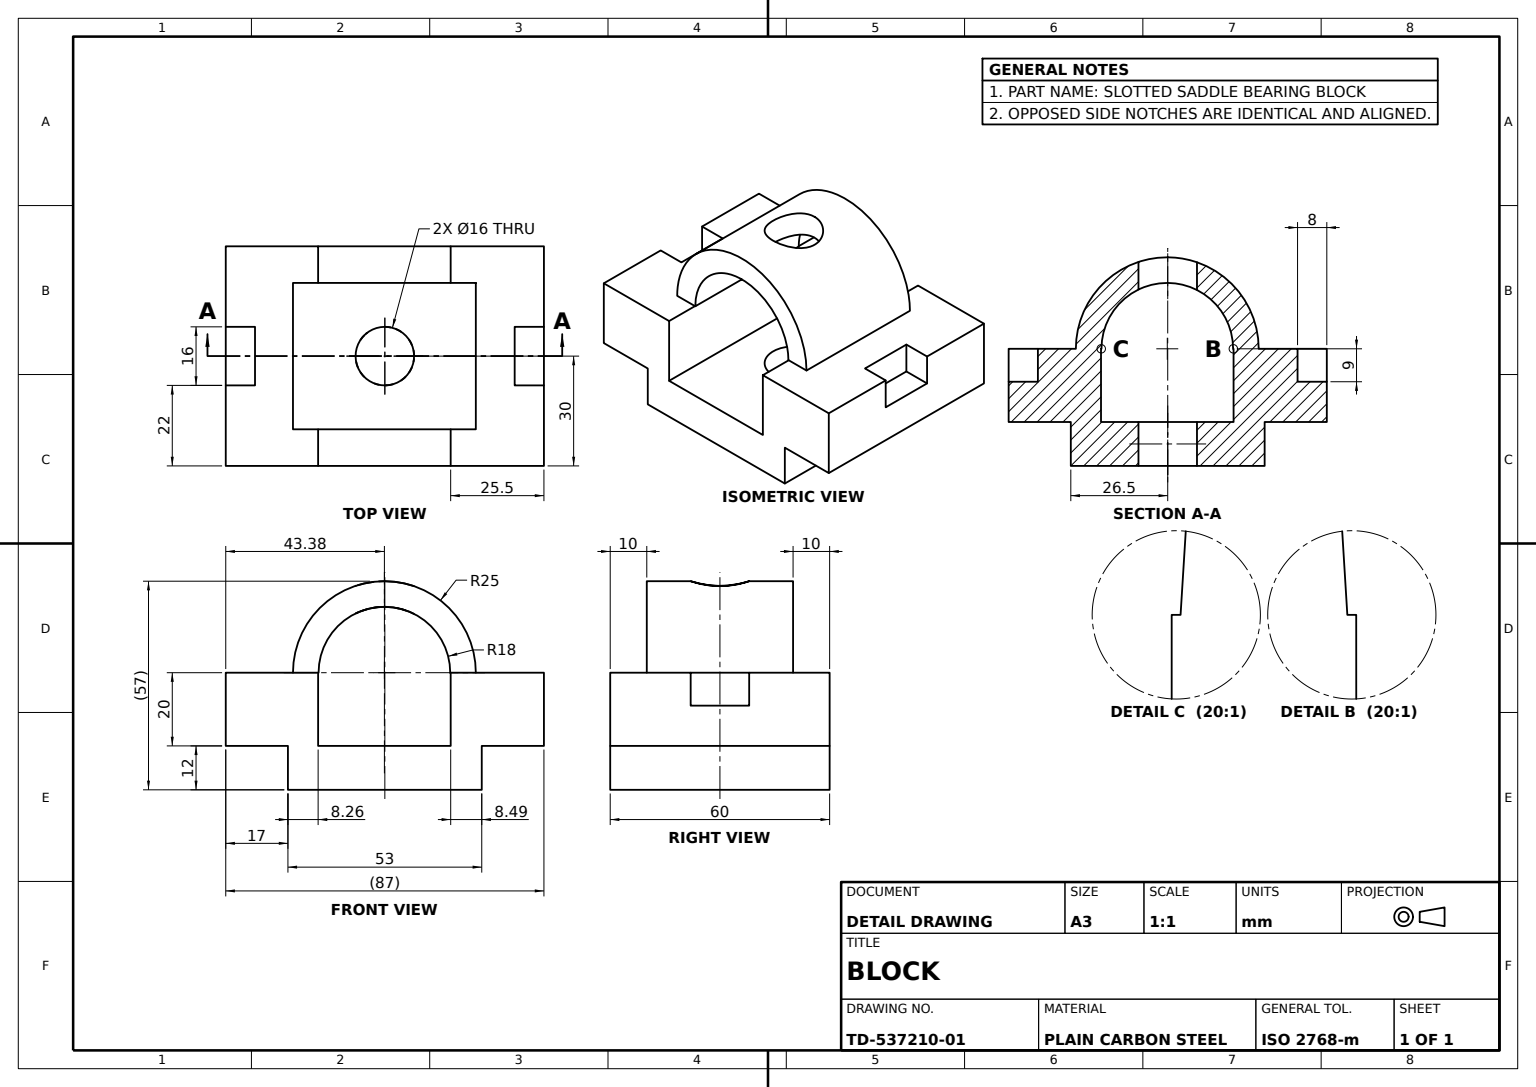
ISO-10303-21;
HEADER;
FILE_DESCRIPTION((''),'2;1');
FILE_NAME('','',(''),(''),'','','');
FILE_SCHEMA(('AUTOMOTIVE_DESIGN'));
ENDSEC;
DATA;
#1=APPLICATION_CONTEXT('');
#2=PRODUCT_CONTEXT('',#1,'mechanical');
#3=PRODUCT('','','',(#2));
#4=PRODUCT_DEFINITION_FORMATION('','',#3);
#5=PRODUCT_DEFINITION_CONTEXT('',#1,'design');
#6=PRODUCT_DEFINITION('','',#4,#5);
#7=PRODUCT_DEFINITION_SHAPE('','',#6);
#8=(LENGTH_UNIT()NAMED_UNIT(*)SI_UNIT(.MILLI.,.METRE.));
#9=(NAMED_UNIT(*)PLANE_ANGLE_UNIT()SI_UNIT($,.RADIAN.));
#10=(NAMED_UNIT(*)SI_UNIT($,.STERADIAN.)SOLID_ANGLE_UNIT());
#11=UNCERTAINTY_MEASURE_WITH_UNIT(LENGTH_MEASURE(1.E-05),#8,'distance_accuracy_value','');
#12=(GEOMETRIC_REPRESENTATION_CONTEXT(3)GLOBAL_UNCERTAINTY_ASSIGNED_CONTEXT((#11))GLOBAL_UNIT_ASSIGNED_CONTEXT((#8,#9,#10))REPRESENTATION_CONTEXT('',''));
#13=CARTESIAN_POINT('',(8.37856,32.,-10.));
#14=VERTEX_POINT('',#13);
#15=CARTESIAN_POINT('',(44.37856,32.,-10.));
#16=VERTEX_POINT('',#15);
#17=CARTESIAN_POINT('',(26.37856,32.,-10.));
#18=DIRECTION('',(0.,0.,-1.));
#19=DIRECTION('',(1.,0.,0.));
#20=AXIS2_PLACEMENT_3D('',#17,#18,#19);
#21=CIRCLE('',#20,18.);
#22=EDGE_CURVE('',#14,#16,#21,.T.);
#23=ORIENTED_EDGE('',*,*,#22,.F.);
#24=CARTESIAN_POINT('',(8.37856,32.,-50.));
#25=VERTEX_POINT('',#24);
#26=CARTESIAN_POINT('',(8.37856,32.,-60.));
#27=DIRECTION('',(0.,0.,1.));
#28=VECTOR('',#27,1000.);
#29=LINE('',#26,#28);
#30=EDGE_CURVE('',#25,#14,#29,.T.);
#31=ORIENTED_EDGE('',*,*,#30,.F.);
#32=CARTESIAN_POINT('',(44.37856,32.,-50.));
#33=VERTEX_POINT('',#32);
#34=CARTESIAN_POINT('',(26.37856,32.,-50.));
#35=DIRECTION('',(-1.,0.,0.));
#36=AXIS2_PLACEMENT_3D('',#34,#27,#35);
#37=CIRCLE('',#36,18.);
#38=EDGE_CURVE('',#33,#25,#37,.T.);
#39=ORIENTED_EDGE('',*,*,#38,.F.);
#40=CARTESIAN_POINT('',(44.37856,32.,-60.));
#41=LINE('',#40,#28);
#42=EDGE_CURVE('',#33,#16,#41,.T.);
#43=ORIENTED_EDGE('',*,*,#42,.T.);
#44=EDGE_LOOP('',(#23,#31,#39,#43));
#45=FACE_OUTER_BOUND('',#44,.T.);
#46=CARTESIAN_POINT('',(26.5,49.99959,-38.));
#47=VERTEX_POINT('',#46);
#48=CARTESIAN_POINT('',(26.5,49.99959,-22.));
#49=VERTEX_POINT('',#48);
#50=CARTESIAN_POINT('',(25.964246,50.003205,-38.));
#51=CARTESIAN_POINT('',(25.438566,49.982898,-37.946734));
#52=CARTESIAN_POINT('',(24.664285,49.920053,-37.790986));
#53=CARTESIAN_POINT('',(24.408581,49.893695,-37.726328));
#54=CARTESIAN_POINT('',(23.902002,49.830642,-37.571036));
#55=CARTESIAN_POINT('',(23.652448,49.794054,-37.480648));
#56=CARTESIAN_POINT('',(22.92738,49.672847,-37.177116));
#57=CARTESIAN_POINT('',(22.469997,49.576171,-36.930418));
#58=CARTESIAN_POINT('',(21.821165,49.414931,-36.494337));
#59=CARTESIAN_POINT('',(21.610763,49.358325,-36.337397));
#60=CARTESIAN_POINT('',(21.21062,49.243425,-36.00747));
#61=CARTESIAN_POINT('',(21.019775,49.184877,-35.83382));
#62=CARTESIAN_POINT('',(20.655906,49.067155,-35.469268));
#63=CARTESIAN_POINT('',(20.482883,49.00798,-35.278366));
#64=CARTESIAN_POINT('',(20.154622,48.890618,-34.878834));
#65=CARTESIAN_POINT('',(19.998702,48.832161,-34.669158));
#66=CARTESIAN_POINT('',(19.563582,48.662921,-34.019669));
#67=CARTESIAN_POINT('',(19.318756,48.559201,-33.563715));
#68=CARTESIAN_POINT('',(19.018105,48.426676,-32.844087));
#69=CARTESIAN_POINT('',(18.929076,48.386349,-32.598217));
#70=CARTESIAN_POINT('',(18.77433,48.315114,-32.093715));
#71=CARTESIAN_POINT('',(18.708786,48.284283,-31.83484));
#72=CARTESIAN_POINT('',(18.552801,48.210205,-31.058601));
#73=CARTESIAN_POINT('',(18.500365,48.184377,-30.535115));
#74=CARTESIAN_POINT('',(18.49982,48.184111,-29.74068));
#75=CARTESIAN_POINT('',(18.512954,48.190525,-29.472639));
#76=CARTESIAN_POINT('',(18.565752,48.216069,-28.9423));
#77=CARTESIAN_POINT('',(18.605134,48.235059,-28.680768));
#78=CARTESIAN_POINT('',(18.708931,48.284351,-28.164645));
#79=CARTESIAN_POINT('',(18.773349,48.314654,-27.910055));
#80=CARTESIAN_POINT('',(18.927099,48.385448,-27.407668));
#81=CARTESIAN_POINT('',(19.016884,48.426139,-27.158821));
#82=CARTESIAN_POINT('',(19.32139,48.560361,-26.430008));
#83=CARTESIAN_POINT('',(19.567938,48.664672,-25.973231));
#84=CARTESIAN_POINT('',(20.145148,48.889063,-25.112852));
#85=CARTESIAN_POINT('',(20.479053,49.010081,-24.707135));
#86=CARTESIAN_POINT('',(21.208844,49.2459,-23.977552));
#87=CARTESIAN_POINT('',(21.606618,49.361664,-23.649682));
#88=CARTESIAN_POINT('',(22.255691,49.522889,-23.213707));
#89=CARTESIAN_POINT('',(22.481555,49.574655,-23.077555));
#90=CARTESIAN_POINT('',(22.941399,49.670345,-22.830306));
#91=CARTESIAN_POINT('',(23.176497,49.714574,-22.718369));
#92=CARTESIAN_POINT('',(23.897426,49.834837,-22.417263));
#93=CARTESIAN_POINT('',(24.399315,49.89856,-22.262283));
#94=CARTESIAN_POINT('',(25.446339,49.983516,-22.051733));
#95=CARTESIAN_POINT('',(25.972085,50.003152,-22.));
#96=B_SPLINE_CURVE_WITH_KNOTS('',3,(#46,#50,#51,#52,#53,#54,#55,#56,#57,#58,#59,#60,#61,#62,#63,#64,#65,#66,#67,#68,#69,#70,#71,#72,#73,#74,#75,#76,#77,#78,#79,#80,#81,#82,#83,#84,#85,#86,#87,#88,#89,#90,#91,#92,#93,#94,#95,#48),.UNSPECIFIED.,.F.,.F.,(4,2,2,2,2,2,2,2,2,2,2,2,2,2,2,2,2,2,2,2,2,2,2,4),(0.,0.001583136,0.002374704,0.003166272,0.004749408,0.005540976,0.006332543,0.007124111,0.007915679,0.009498815,0.010290383,0.011081951,0.012665087,0.013456655,0.014248223,0.015039791,0.015831359,0.017414494,0.01899763,0.020580766,0.021372334,0.022163902,0.023747038,0.025330174),.UNSPECIFIED.);
#97=EDGE_CURVE('',#47,#49,#96,.T.);
#98=ORIENTED_EDGE('',*,*,#97,.T.);
#99=CARTESIAN_POINT('',(26.764064,49.997809,-22.));
#100=CARTESIAN_POINT('',(27.028674,49.990215,-22.013041));
#101=CARTESIAN_POINT('',(27.559017,49.963213,-22.065928));
#102=CARTESIAN_POINT('',(27.824003,49.943758,-22.105896));
#103=CARTESIAN_POINT('',(28.601301,49.869818,-22.262817));
#104=CARTESIAN_POINT('',(29.102564,49.799515,-22.416925));
#105=CARTESIAN_POINT('',(29.830027,49.667714,-22.721263));
#106=CARTESIAN_POINT('',(30.068623,49.619273,-22.835297));
#107=CARTESIAN_POINT('',(30.527777,49.51683,-23.082988));
#108=CARTESIAN_POINT('',(30.749676,49.462605,-23.217147));
#109=CARTESIAN_POINT('',(31.178754,49.349564,-23.505687));
#110=CARTESIAN_POINT('',(31.385933,49.290744,-23.660069));
#111=CARTESIAN_POINT('',(31.785742,49.169915,-23.989343));
#112=CARTESIAN_POINT('',(31.979206,49.107603,-24.16516));
#113=CARTESIAN_POINT('',(32.527994,48.921398,-24.714975));
#114=CARTESIAN_POINT('',(32.854204,48.797694,-25.112178));
#115=CARTESIAN_POINT('',(33.429913,48.564266,-25.969738));
#116=CARTESIAN_POINT('',(33.680853,48.453733,-26.435349));
#117=CARTESIAN_POINT('',(34.082504,48.269544,-27.396727));
#118=CARTESIAN_POINT('',(34.236223,48.194777,-27.895252));
#119=CARTESIAN_POINT('',(34.393423,48.117239,-28.671973));
#120=CARTESIAN_POINT('',(34.433605,48.097116,-28.937576));
#121=CARTESIAN_POINT('',(34.486676,48.070449,-29.467229));
#122=CARTESIAN_POINT('',(34.499857,48.063765,-29.731661));
#123=CARTESIAN_POINT('',(34.500282,48.06355,-30.523798));
#124=CARTESIAN_POINT('',(34.448308,48.090147,-31.052725));
#125=CARTESIAN_POINT('',(34.238524,48.193661,-32.097398));
#126=CARTESIAN_POINT('',(34.08416,48.268767,-32.59878));
#127=CARTESIAN_POINT('',(33.681598,48.453409,-33.563396));
#128=CARTESIAN_POINT('',(33.430864,48.563868,-34.028716));
#129=CARTESIAN_POINT('',(32.854504,48.797585,-34.887505));
#130=CARTESIAN_POINT('',(32.527462,48.921632,-35.285848));
#131=CARTESIAN_POINT('',(31.792354,49.170948,-36.02175));
#132=CARTESIAN_POINT('',(31.392307,49.293306,-36.350717));
#133=CARTESIAN_POINT('',(30.749986,49.462522,-36.782639));
#134=CARTESIAN_POINT('',(30.528437,49.51667,-36.916618));
#135=CARTESIAN_POINT('',(30.069763,49.61903,-37.164126));
#136=CARTESIAN_POINT('',(29.831126,49.6675,-37.278238));
#137=CARTESIAN_POINT('',(29.103381,49.799395,-37.582811));
#138=CARTESIAN_POINT('',(28.603202,49.869504,-37.736487));
#139=CARTESIAN_POINT('',(27.829887,49.943263,-37.893071));
#140=CARTESIAN_POINT('',(27.56825,49.962612,-37.932853));
#141=CARTESIAN_POINT('',(27.036837,49.989927,-37.986434));
#142=CARTESIAN_POINT('',(26.767985,49.997782,-38.));
#143=B_SPLINE_CURVE_WITH_KNOTS('',3,(#48,#99,#100,#101,#102,#103,#104,#105,#106,#107,#108,#109,#110,#111,#112,#113,#114,#115,#116,#117,#118,#119,#120,#121,#122,#123,#124,#125,#126,#127,#128,#129,#130,#131,#132,#133,#134,#135,#136,#137,#138,#139,#140,#141,#142,#46),.UNSPECIFIED.,.F.,.F.,(4,2,2,2,2,2,2,2,2,2,2,2,2,2,2,2,2,2,2,2,2,2,4),(0.025330174,0.02612206,0.026913946,0.028497719,0.029289605,0.030081491,0.030873378,0.031665264,0.033249036,0.034832809,0.036416582,0.037208468,0.038000354,0.039584127,0.041167899,0.042751672,0.044335444,0.045919217,0.046711103,0.047502989,0.049086762,0.049878648,0.050670534),.UNSPECIFIED.);
#144=EDGE_CURVE('',#49,#47,#143,.T.);
#145=ORIENTED_EDGE('',*,*,#144,.T.);
#146=EDGE_LOOP('',(#98,#145));
#147=FACE_BOUND('',#146,.T.);
#148=CARTESIAN_POINT('',(26.37856,32.,-60.));
#149=AXIS2_PLACEMENT_3D('',#148,#27,#19);
#150=CYLINDRICAL_SURFACE('',#149,18.);
#151=ADVANCED_FACE('',(#45,#147),#150,.F.);
#152=CARTESIAN_POINT('',(8.25712,32.,-10.));
#153=VERTEX_POINT('',#152);
#154=CARTESIAN_POINT('',(1.37856,32.,-10.));
#155=VERTEX_POINT('',#154);
#156=CARTESIAN_POINT('',(0.,32.,-10.));
#157=VECTOR('',#35,1000.);
#158=LINE('',#156,#157);
#159=EDGE_CURVE('',#153,#155,#158,.T.);
#160=ORIENTED_EDGE('',*,*,#159,.T.);
#161=CARTESIAN_POINT('',(1.37856,32.,-50.));
#162=VERTEX_POINT('',#161);
#163=CARTESIAN_POINT('',(1.37856,32.,-60.));
#164=LINE('',#163,#28);
#165=EDGE_CURVE('',#162,#155,#164,.T.);
#166=ORIENTED_EDGE('',*,*,#165,.F.);
#167=CARTESIAN_POINT('',(8.25712,32.,-50.));
#168=VERTEX_POINT('',#167);
#169=LINE('',#24,#157);
#170=EDGE_CURVE('',#168,#162,#169,.T.);
#171=ORIENTED_EDGE('',*,*,#170,.F.);
#172=CARTESIAN_POINT('',(8.25712,32.,-60.));
#173=VERTEX_POINT('',#172);
#174=LINE('',#172,#28);
#175=EDGE_CURVE('',#173,#168,#174,.T.);
#176=ORIENTED_EDGE('',*,*,#175,.F.);
#177=CARTESIAN_POINT('',(-17.,32.,-60.));
#178=VERTEX_POINT('',#177);
#179=LINE('',#177,#157);
#180=EDGE_CURVE('',#173,#178,#179,.T.);
#181=ORIENTED_EDGE('',*,*,#180,.T.);
#182=CARTESIAN_POINT('',(-17.,32.,-38.));
#183=VERTEX_POINT('',#182);
#184=LINE('',#177,#28);
#185=EDGE_CURVE('',#178,#183,#184,.T.);
#186=ORIENTED_EDGE('',*,*,#185,.T.);
#187=CARTESIAN_POINT('',(-9.,32.,-38.));
#188=VERTEX_POINT('',#187);
#189=LINE('',#182,#157);
#190=EDGE_CURVE('',#188,#183,#189,.T.);
#191=ORIENTED_EDGE('',*,*,#190,.F.);
#192=CARTESIAN_POINT('',(-9.,32.,-22.));
#193=VERTEX_POINT('',#192);
#194=VECTOR('',#18,1000.);
#195=LINE('',#187,#194);
#196=EDGE_CURVE('',#193,#188,#195,.T.);
#197=ORIENTED_EDGE('',*,*,#196,.F.);
#198=CARTESIAN_POINT('',(-17.,32.,-22.));
#199=VERTEX_POINT('',#198);
#200=VECTOR('',#19,1000.);
#201=LINE('',#192,#200);
#202=EDGE_CURVE('',#199,#193,#201,.T.);
#203=ORIENTED_EDGE('',*,*,#202,.F.);
#204=CARTESIAN_POINT('',(-17.,32.,0.));
#205=VERTEX_POINT('',#204);
#206=EDGE_CURVE('',#199,#205,#184,.T.);
#207=ORIENTED_EDGE('',*,*,#206,.T.);
#208=CARTESIAN_POINT('',(8.25712,32.,0.));
#209=VERTEX_POINT('',#208);
#210=LINE('',#204,#157);
#211=EDGE_CURVE('',#209,#205,#210,.T.);
#212=ORIENTED_EDGE('',*,*,#211,.F.);
#213=EDGE_CURVE('',#153,#209,#174,.T.);
#214=ORIENTED_EDGE('',*,*,#213,.F.);
#215=EDGE_LOOP('',(#160,#166,#171,#176,#181,#186,#191,#197,#203,#207,#212,#214));
#216=FACE_OUTER_BOUND('',#215,.T.);
#217=DIRECTION('',(0.,1.,0.));
#218=AXIS2_PLACEMENT_3D('',#177,#217,#27);
#219=PLANE('',#218);
#220=ADVANCED_FACE('',(#216),#219,.T.);
#221=CARTESIAN_POINT('',(53.,0.,0.));
#222=VERTEX_POINT('',#221);
#223=CARTESIAN_POINT('',(53.,12.,0.));
#224=VERTEX_POINT('',#223);
#225=VECTOR('',#217,1000.);
#226=LINE('',#221,#225);
#227=EDGE_CURVE('',#222,#224,#226,.T.);
#228=ORIENTED_EDGE('',*,*,#227,.T.);
#229=CARTESIAN_POINT('',(70.,12.,0.));
#230=VERTEX_POINT('',#229);
#231=LINE('',#223,#200);
#232=EDGE_CURVE('',#224,#230,#231,.T.);
#233=ORIENTED_EDGE('',*,*,#232,.T.);
#234=CARTESIAN_POINT('',(70.,32.,0.));
#235=VERTEX_POINT('',#234);
#236=LINE('',#234,#225);
#237=EDGE_CURVE('',#230,#235,#236,.T.);
#238=ORIENTED_EDGE('',*,*,#237,.T.);
#239=CARTESIAN_POINT('',(44.5,32.,0.));
#240=VERTEX_POINT('',#239);
#241=LINE('',#239,#157);
#242=EDGE_CURVE('',#235,#240,#241,.T.);
#243=ORIENTED_EDGE('',*,*,#242,.T.);
#244=CARTESIAN_POINT('',(44.508364,12.,0.));
#245=VERTEX_POINT('',#244);
#246=DIRECTION('',(0.00041821,-0.999999913,0.));
#247=VECTOR('',#246,1000.);
#248=LINE('',#244,#247);
#249=EDGE_CURVE('',#240,#245,#248,.T.);
#250=ORIENTED_EDGE('',*,*,#249,.T.);
#251=CARTESIAN_POINT('',(8.25712,12.,0.));
#252=VERTEX_POINT('',#251);
#253=LINE('',#251,#157);
#254=EDGE_CURVE('',#245,#252,#253,.T.);
#255=ORIENTED_EDGE('',*,*,#254,.T.);
#256=LINE('',#208,#225);
#257=EDGE_CURVE('',#252,#209,#256,.T.);
#258=ORIENTED_EDGE('',*,*,#257,.T.);
#259=ORIENTED_EDGE('',*,*,#211,.T.);
#260=CARTESIAN_POINT('',(-17.,12.,0.));
#261=VERTEX_POINT('',#260);
#262=DIRECTION('',(0.,-1.,0.));
#263=VECTOR('',#262,1000.);
#264=LINE('',#260,#263);
#265=EDGE_CURVE('',#205,#261,#264,.T.);
#266=ORIENTED_EDGE('',*,*,#265,.T.);
#267=CARTESIAN_POINT('',(0.,12.,0.));
#268=VERTEX_POINT('',#267);
#269=LINE('',#267,#200);
#270=EDGE_CURVE('',#261,#268,#269,.T.);
#271=ORIENTED_EDGE('',*,*,#270,.T.);
#272=CARTESIAN_POINT('',(0.,0.,0.));
#273=VERTEX_POINT('',#272);
#274=LINE('',#272,#263);
#275=EDGE_CURVE('',#268,#273,#274,.T.);
#276=ORIENTED_EDGE('',*,*,#275,.T.);
#277=LINE('',#272,#200);
#278=EDGE_CURVE('',#273,#222,#277,.T.);
#279=ORIENTED_EDGE('',*,*,#278,.T.);
#280=EDGE_LOOP('',(#228,#233,#238,#243,#250,#255,#258,#259,#266,#271,#276,#279));
#281=FACE_OUTER_BOUND('',#280,.T.);
#282=AXIS2_PLACEMENT_3D('',#272,#27,#19);
#283=PLANE('',#282);
#284=ADVANCED_FACE('',(#281),#283,.T.);
#285=CARTESIAN_POINT('',(0.,0.,-60.));
#286=VERTEX_POINT('',#285);
#287=LINE('',#285,#28);
#288=EDGE_CURVE('',#286,#273,#287,.T.);
#289=ORIENTED_EDGE('',*,*,#288,.T.);
#290=ORIENTED_EDGE('',*,*,#275,.F.);
#291=CARTESIAN_POINT('',(0.,12.,-60.));
#292=VERTEX_POINT('',#291);
#293=LINE('',#291,#28);
#294=EDGE_CURVE('',#292,#268,#293,.T.);
#295=ORIENTED_EDGE('',*,*,#294,.F.);
#296=LINE('',#285,#263);
#297=EDGE_CURVE('',#292,#286,#296,.T.);
#298=ORIENTED_EDGE('',*,*,#297,.T.);
#299=EDGE_LOOP('',(#289,#290,#295,#298));
#300=FACE_OUTER_BOUND('',#299,.T.);
#301=AXIS2_PLACEMENT_3D('',#285,#35,#27);
#302=PLANE('',#301);
#303=ADVANCED_FACE('',(#300),#302,.T.);
#304=CARTESIAN_POINT('',(-17.,23.,-38.));
#305=VERTEX_POINT('',#304);
#306=LINE('',#304,#225);
#307=EDGE_CURVE('',#305,#183,#306,.T.);
#308=ORIENTED_EDGE('',*,*,#307,.F.);
#309=CARTESIAN_POINT('',(-9.,23.,-38.));
#310=VERTEX_POINT('',#309);
#311=LINE('',#304,#157);
#312=EDGE_CURVE('',#310,#305,#311,.T.);
#313=ORIENTED_EDGE('',*,*,#312,.F.);
#314=LINE('',#309,#225);
#315=EDGE_CURVE('',#310,#188,#314,.T.);
#316=ORIENTED_EDGE('',*,*,#315,.T.);
#317=ORIENTED_EDGE('',*,*,#190,.T.);
#318=EDGE_LOOP('',(#308,#313,#316,#317));
#319=FACE_OUTER_BOUND('',#318,.T.);
#320=AXIS2_PLACEMENT_3D('',#304,#18,#35);
#321=PLANE('',#320);
#322=ADVANCED_FACE('',(#319),#321,.F.);
#323=CARTESIAN_POINT('',(44.5,32.,-50.));
#324=VERTEX_POINT('',#323);
#325=CARTESIAN_POINT('',(51.37856,32.,-50.));
#326=LINE('',#325,#157);
#327=EDGE_CURVE('',#324,#33,#326,.T.);
#328=ORIENTED_EDGE('',*,*,#327,.F.);
#329=CARTESIAN_POINT('',(44.5,32.,-10.));
#330=VERTEX_POINT('',#329);
#331=CARTESIAN_POINT('',(44.5,32.,-60.));
#332=LINE('',#331,#28);
#333=EDGE_CURVE('',#324,#330,#332,.T.);
#334=ORIENTED_EDGE('',*,*,#333,.T.);
#335=LINE('',#156,#200);
#336=EDGE_CURVE('',#16,#330,#335,.T.);
#337=ORIENTED_EDGE('',*,*,#336,.F.);
#338=ORIENTED_EDGE('',*,*,#42,.F.);
#339=EDGE_LOOP('',(#328,#334,#337,#338));
#340=FACE_OUTER_BOUND('',#339,.T.);
#341=CARTESIAN_POINT('',(0.,32.,-60.));
#342=AXIS2_PLACEMENT_3D('',#341,#217,#27);
#343=PLANE('',#342);
#344=ADVANCED_FACE('',(#340),#343,.F.);
#345=CARTESIAN_POINT('',(-9.,23.,-22.));
#346=VERTEX_POINT('',#345);
#347=LINE('',#345,#225);
#348=EDGE_CURVE('',#346,#193,#347,.T.);
#349=ORIENTED_EDGE('',*,*,#348,.T.);
#350=ORIENTED_EDGE('',*,*,#196,.T.);
#351=ORIENTED_EDGE('',*,*,#315,.F.);
#352=LINE('',#309,#194);
#353=EDGE_CURVE('',#346,#310,#352,.T.);
#354=ORIENTED_EDGE('',*,*,#353,.F.);
#355=EDGE_LOOP('',(#349,#350,#351,#354));
#356=FACE_OUTER_BOUND('',#355,.T.);
#357=AXIS2_PLACEMENT_3D('',#309,#19,#18);
#358=PLANE('',#357);
#359=ADVANCED_FACE('',(#356),#358,.F.);
#360=CARTESIAN_POINT('',(62.,23.,-22.));
#361=VERTEX_POINT('',#360);
#362=CARTESIAN_POINT('',(70.,23.,-22.));
#363=VERTEX_POINT('',#362);
#364=LINE('',#360,#200);
#365=EDGE_CURVE('',#361,#363,#364,.T.);
#366=ORIENTED_EDGE('',*,*,#365,.F.);
#367=CARTESIAN_POINT('',(62.,32.,-22.));
#368=VERTEX_POINT('',#367);
#369=LINE('',#360,#225);
#370=EDGE_CURVE('',#361,#368,#369,.T.);
#371=ORIENTED_EDGE('',*,*,#370,.T.);
#372=CARTESIAN_POINT('',(70.,32.,-22.));
#373=VERTEX_POINT('',#372);
#374=LINE('',#367,#200);
#375=EDGE_CURVE('',#368,#373,#374,.T.);
#376=ORIENTED_EDGE('',*,*,#375,.T.);
#377=LINE('',#362,#225);
#378=EDGE_CURVE('',#363,#373,#377,.T.);
#379=ORIENTED_EDGE('',*,*,#378,.F.);
#380=EDGE_LOOP('',(#366,#371,#376,#379));
#381=FACE_OUTER_BOUND('',#380,.T.);
#382=AXIS2_PLACEMENT_3D('',#360,#27,#19);
#383=PLANE('',#382);
#384=ADVANCED_FACE('',(#381),#383,.F.);
#385=CARTESIAN_POINT('',(26.5,56.999705,-38.));
#386=VERTEX_POINT('',#385);
#387=CARTESIAN_POINT('',(26.5,100.,-38.));
#388=LINE('',#387,#263);
#389=EDGE_CURVE('',#386,#47,#388,.T.);
#390=ORIENTED_EDGE('',*,*,#389,.F.);
#391=CARTESIAN_POINT('',(26.5,56.999705,-22.));
#392=VERTEX_POINT('',#391);
#393=CARTESIAN_POINT('',(25.967838,57.00229,-38.));
#394=CARTESIAN_POINT('',(25.445152,56.987867,-37.947435));
#395=CARTESIAN_POINT('',(24.674623,56.943191,-37.793369));
#396=CARTESIAN_POINT('',(24.420046,56.924453,-37.729382));
#397=CARTESIAN_POINT('',(23.915495,56.879659,-37.575611));
#398=CARTESIAN_POINT('',(23.665721,56.853568,-37.485688));
#399=CARTESIAN_POINT('',(22.940035,56.767194,-37.183405));
#400=CARTESIAN_POINT('',(22.481671,56.698343,-36.937252));
#401=CARTESIAN_POINT('',(21.831174,56.583933,-36.501551));
#402=CARTESIAN_POINT('',(21.619519,56.543715,-36.344225));
#403=CARTESIAN_POINT('',(21.215883,56.461994,-36.012187));
#404=CARTESIAN_POINT('',(21.023549,56.420465,-35.837434));
#405=CARTESIAN_POINT('',(20.474092,56.295645,-35.287443));
#406=CARTESIAN_POINT('',(20.144221,56.212079,-34.88675));
#407=CARTESIAN_POINT('',(19.559498,56.053942,-34.013188));
#408=CARTESIAN_POINT('',(19.313689,55.981894,-33.553568));
#409=CARTESIAN_POINT('',(19.013782,55.890813,-32.832715));
#410=CARTESIAN_POINT('',(18.925281,55.863258,-32.58702));
#411=CARTESIAN_POINT('',(18.771847,55.814793,-32.084394));
#412=CARTESIAN_POINT('',(18.706736,55.793824,-31.826069));
#413=CARTESIAN_POINT('',(18.55178,55.74349,-31.050593));
#414=CARTESIAN_POINT('',(18.500244,55.726191,-30.529299));
#415=CARTESIAN_POINT('',(18.499757,55.726029,-29.478114));
#416=CARTESIAN_POINT('',(18.552643,55.743773,-28.944208));
#417=CARTESIAN_POINT('',(18.758559,55.810655,-27.915468));
#418=CARTESIAN_POINT('',(18.910816,55.859537,-27.415068));
#419=CARTESIAN_POINT('',(19.214228,55.951691,-26.685348));
#420=CARTESIAN_POINT('',(19.327484,55.985388,-26.447097));
#421=CARTESIAN_POINT('',(19.574287,56.056566,-25.987194));
#422=CARTESIAN_POINT('',(19.708278,56.094185,-25.764445));
#423=CARTESIAN_POINT('',(19.997197,56.172311,-25.332992));
#424=CARTESIAN_POINT('',(20.152125,56.21282,-25.124288));
#425=CARTESIAN_POINT('',(20.483338,56.295586,-24.720998));
#426=CARTESIAN_POINT('',(20.660412,56.338006,-24.525772));
#427=CARTESIAN_POINT('',(21.213607,56.46357,-23.972902));
#428=CARTESIAN_POINT('',(21.613981,56.545701,-23.644087));
#429=CARTESIAN_POINT('',(22.47858,56.69783,-23.064656));
#430=CARTESIAN_POINT('',(22.947108,56.76814,-22.813244));
#431=CARTESIAN_POINT('',(23.911153,56.882675,-22.412486));
#432=CARTESIAN_POINT('',(24.410455,56.927799,-22.259701));
#433=CARTESIAN_POINT('',(25.186509,56.972908,-22.104156));
#434=CARTESIAN_POINT('',(25.450595,56.984151,-22.064742));
#435=CARTESIAN_POINT('',(25.975543,56.99813,-22.012853));
#436=CARTESIAN_POINT('',(26.237852,57.000978,-22.));
#437=B_SPLINE_CURVE_WITH_KNOTS('',3,(#385,#393,#394,#395,#396,#397,#398,#399,#400,#401,#402,#403,#404,#405,#406,#407,#408,#409,#410,#411,#412,#413,#414,#415,#416,#417,#418,#419,#420,#421,#422,#423,#424,#425,#426,#427,#428,#429,#430,#431,#432,#433,#434,#435,#436,#391),.UNSPECIFIED.,.F.,.F.,(4,2,2,2,2,2,2,2,2,2,2,2,2,2,2,2,2,2,2,2,2,2,4),(0.,0.001573119,0.002359679,0.003146238,0.004719358,0.005505917,0.006292477,0.007865596,0.009438715,0.010225275,0.011011834,0.012584953,0.014158073,0.015731192,0.016517751,0.017304311,0.01809087,0.01887743,0.020450549,0.022023668,0.023596788,0.024383347,0.025169907),.UNSPECIFIED.);
#438=EDGE_CURVE('',#386,#392,#437,.T.);
#439=ORIENTED_EDGE('',*,*,#438,.T.);
#440=CARTESIAN_POINT('',(26.5,100.,-22.));
#441=LINE('',#440,#263);
#442=EDGE_CURVE('',#392,#49,#441,.T.);
#443=ORIENTED_EDGE('',*,*,#442,.T.);
#444=ORIENTED_EDGE('',*,*,#97,.F.);
#445=EDGE_LOOP('',(#390,#439,#443,#444));
#446=FACE_OUTER_BOUND('',#445,.T.);
#447=CARTESIAN_POINT('',(26.5,100.,-30.));
#448=AXIS2_PLACEMENT_3D('',#447,#262,#18);
#449=CYLINDRICAL_SURFACE('',#448,8.);
#450=ADVANCED_FACE('',(#446),#449,.F.);
#451=VERTEX_POINT('',#325);
#452=CARTESIAN_POINT('',(51.37856,32.,-10.));
#453=VERTEX_POINT('',#452);
#454=CARTESIAN_POINT('',(51.37856,32.,-60.));
#455=LINE('',#454,#28);
#456=EDGE_CURVE('',#451,#453,#455,.T.);
#457=ORIENTED_EDGE('',*,*,#456,.T.);
#458=EDGE_CURVE('',#330,#453,#335,.T.);
#459=ORIENTED_EDGE('',*,*,#458,.F.);
#460=EDGE_CURVE('',#330,#240,#332,.T.);
#461=ORIENTED_EDGE('',*,*,#460,.T.);
#462=ORIENTED_EDGE('',*,*,#242,.F.);
#463=CARTESIAN_POINT('',(70.,32.,-60.));
#464=LINE('',#463,#28);
#465=EDGE_CURVE('',#373,#235,#464,.T.);
#466=ORIENTED_EDGE('',*,*,#465,.F.);
#467=ORIENTED_EDGE('',*,*,#375,.F.);
#468=CARTESIAN_POINT('',(62.,32.,-38.));
#469=VERTEX_POINT('',#468);
#470=LINE('',#468,#28);
#471=EDGE_CURVE('',#469,#368,#470,.T.);
#472=ORIENTED_EDGE('',*,*,#471,.F.);
#473=CARTESIAN_POINT('',(70.,32.,-38.));
#474=VERTEX_POINT('',#473);
#475=LINE('',#473,#157);
#476=EDGE_CURVE('',#474,#469,#475,.T.);
#477=ORIENTED_EDGE('',*,*,#476,.F.);
#478=VERTEX_POINT('',#463);
#479=EDGE_CURVE('',#478,#474,#464,.T.);
#480=ORIENTED_EDGE('',*,*,#479,.F.);
#481=VERTEX_POINT('',#331);
#482=LINE('',#331,#157);
#483=EDGE_CURVE('',#478,#481,#482,.T.);
#484=ORIENTED_EDGE('',*,*,#483,.T.);
#485=EDGE_CURVE('',#481,#324,#332,.T.);
#486=ORIENTED_EDGE('',*,*,#485,.T.);
#487=EDGE_CURVE('',#451,#324,#326,.T.);
#488=ORIENTED_EDGE('',*,*,#487,.F.);
#489=EDGE_LOOP('',(#457,#459,#461,#462,#466,#467,#472,#477,#480,#484,#486,#488));
#490=FACE_OUTER_BOUND('',#489,.T.);
#491=AXIS2_PLACEMENT_3D('',#331,#217,#27);
#492=PLANE('',#491);
#493=ADVANCED_FACE('',(#490),#492,.T.);
#494=ORIENTED_EDGE('',*,*,#22,.T.);
#495=ORIENTED_EDGE('',*,*,#336,.T.);
#496=ORIENTED_EDGE('',*,*,#458,.T.);
#497=AXIS2_PLACEMENT_3D('',#17,#27,#19);
#498=CIRCLE('',#497,25.);
#499=EDGE_CURVE('',#453,#155,#498,.T.);
#500=ORIENTED_EDGE('',*,*,#499,.T.);
#501=ORIENTED_EDGE('',*,*,#159,.F.);
#502=EDGE_CURVE('',#14,#153,#158,.T.);
#503=ORIENTED_EDGE('',*,*,#502,.F.);
#504=EDGE_LOOP('',(#494,#495,#496,#500,#501,#503));
#505=FACE_OUTER_BOUND('',#504,.T.);
#506=CARTESIAN_POINT('',(0.,0.,-10.));
#507=AXIS2_PLACEMENT_3D('',#506,#27,#19);
#508=PLANE('',#507);
#509=ADVANCED_FACE('',(#505),#508,.T.);
#510=ORIENTED_EDGE('',*,*,#456,.F.);
#511=AXIS2_PLACEMENT_3D('',#34,#18,#35);
#512=CIRCLE('',#511,25.);
#513=EDGE_CURVE('',#162,#451,#512,.T.);
#514=ORIENTED_EDGE('',*,*,#513,.F.);
#515=ORIENTED_EDGE('',*,*,#165,.T.);
#516=ORIENTED_EDGE('',*,*,#499,.F.);
#517=EDGE_LOOP('',(#510,#514,#515,#516));
#518=FACE_OUTER_BOUND('',#517,.T.);
#519=CARTESIAN_POINT('',(26.762267,56.998431,-22.));
#520=CARTESIAN_POINT('',(27.024372,56.993032,-22.012866));
#521=CARTESIAN_POINT('',(27.548255,56.973997,-22.064608));
#522=CARTESIAN_POINT('',(27.811411,56.96026,-22.103783));
#523=CARTESIAN_POINT('',(28.589956,56.907436,-22.259698));
#524=CARTESIAN_POINT('',(29.090191,56.857265,-22.412913));
#525=CARTESIAN_POINT('',(30.05499,56.732983,-22.814248));
#526=CARTESIAN_POINT('',(30.52293,56.658008,-23.065546));
#527=CARTESIAN_POINT('',(31.387099,56.497096,-23.644932));
#528=CARTESIAN_POINT('',(31.787614,56.410779,-23.973915));
#529=CARTESIAN_POINT('',(32.341365,56.279229,-24.527651));
#530=CARTESIAN_POINT('',(32.518107,56.234997,-24.722679));
#531=CARTESIAN_POINT('',(32.848398,56.14892,-25.125004));
#532=CARTESIAN_POINT('',(33.002972,56.106837,-25.333255));
#533=CARTESIAN_POINT('',(33.291359,56.025729,-25.763893));
#534=CARTESIAN_POINT('',(33.425171,55.986701,-25.986281));
#535=CARTESIAN_POINT('',(33.671757,55.91288,-26.445589));
#536=CARTESIAN_POINT('',(33.78494,55.877957,-26.683508));
#537=CARTESIAN_POINT('',(34.08867,55.782331,-27.413509));
#538=CARTESIAN_POINT('',(34.240815,55.731767,-27.913446));
#539=CARTESIAN_POINT('',(34.395218,55.679868,-28.683178));
#540=CARTESIAN_POINT('',(34.434291,55.666558,-28.943081));
#541=CARTESIAN_POINT('',(34.486798,55.64862,-29.469804));
#542=CARTESIAN_POINT('',(34.500008,55.644071,-29.736534));
#543=CARTESIAN_POINT('',(34.499985,55.644079,-30.527626));
#544=CARTESIAN_POINT('',(34.448324,55.66201,-31.049497));
#545=CARTESIAN_POINT('',(34.293712,55.71399,-31.824111));
#546=CARTESIAN_POINT('',(34.228727,55.735657,-32.08236));
#547=CARTESIAN_POINT('',(34.074929,55.785972,-32.586483));
#548=CARTESIAN_POINT('',(33.986197,55.814594,-32.832826));
#549=CARTESIAN_POINT('',(33.685511,55.909258,-33.555369));
#550=CARTESIAN_POINT('',(33.438223,55.984437,-34.017007));
#551=CARTESIAN_POINT('',(32.854151,56.14868,-34.888766));
#552=CARTESIAN_POINT('',(32.524467,56.235712,-35.289095));
#553=CARTESIAN_POINT('',(31.974731,56.366336,-35.83905));
#554=CARTESIAN_POINT('',(31.782211,56.409901,-36.013877));
#555=CARTESIAN_POINT('',(31.377944,56.495895,-36.34619));
#556=CARTESIAN_POINT('',(31.166845,56.538149,-36.502948));
#557=CARTESIAN_POINT('',(30.517833,56.658875,-36.937444));
#558=CARTESIAN_POINT('',(30.060391,56.732192,-37.183137));
#559=CARTESIAN_POINT('',(29.335836,56.825669,-37.485085));
#560=CARTESIAN_POINT('',(29.086445,56.854209,-37.574957));
#561=CARTESIAN_POINT('',(28.581514,56.904043,-37.728969));
#562=CARTESIAN_POINT('',(28.326748,56.925307,-37.793055));
#563=CARTESIAN_POINT('',(27.555645,56.977589,-37.947356));
#564=CARTESIAN_POINT('',(27.032404,56.997119,-38.));
#565=B_SPLINE_CURVE_WITH_KNOTS('',3,(#391,#519,#520,#521,#522,#523,#524,#525,#526,#527,#528,#529,#530,#531,#532,#533,#534,#535,#536,#537,#538,#539,#540,#541,#542,#543,#544,#545,#546,#547,#548,#549,#550,#551,#552,#553,#554,#555,#556,#557,#558,#559,#560,#561,#562,#563,#564,#385),.UNSPECIFIED.,.F.,.F.,(4,2,2,2,2,2,2,2,2,2,2,2,2,2,2,2,2,2,2,2,2,2,2,4),(0.025169907,0.025956825,0.026743743,0.028317579,0.029891415,0.03146525,0.032252168,0.033039086,0.033826004,0.034612922,0.036186758,0.036973676,0.037760594,0.03933443,0.040121348,0.040908266,0.042482102,0.044055938,0.044842856,0.045629774,0.04720361,0.047990528,0.048777446,0.050351282),.UNSPECIFIED.);
#566=EDGE_CURVE('',#392,#386,#565,.T.);
#567=ORIENTED_EDGE('',*,*,#566,.F.);
#568=ORIENTED_EDGE('',*,*,#438,.F.);
#569=EDGE_LOOP('',(#567,#568));
#570=FACE_BOUND('',#569,.T.);
#571=CYLINDRICAL_SURFACE('',#149,25.);
#572=ADVANCED_FACE('',(#518,#570),#571,.T.);
#573=ORIENTED_EDGE('',*,*,#144,.F.);
#574=ORIENTED_EDGE('',*,*,#442,.F.);
#575=ORIENTED_EDGE('',*,*,#566,.T.);
#576=ORIENTED_EDGE('',*,*,#389,.T.);
#577=EDGE_LOOP('',(#573,#574,#575,#576));
#578=FACE_OUTER_BOUND('',#577,.T.);
#579=ADVANCED_FACE('',(#578),#449,.F.);
#580=CARTESIAN_POINT('',(26.5,0.,-38.));
#581=VERTEX_POINT('',#580);
#582=CARTESIAN_POINT('',(26.5,0.,-22.));
#583=VERTEX_POINT('',#582);
#584=CARTESIAN_POINT('',(26.5,0.,-30.));
#585=AXIS2_PLACEMENT_3D('',#584,#262,#18);
#586=CIRCLE('',#585,8.);
#587=EDGE_CURVE('',#581,#583,#586,.T.);
#588=ORIENTED_EDGE('',*,*,#587,.T.);
#589=CARTESIAN_POINT('',(26.5,12.,-22.));
#590=VERTEX_POINT('',#589);
#591=EDGE_CURVE('',#590,#583,#441,.T.);
#592=ORIENTED_EDGE('',*,*,#591,.F.);
#593=CARTESIAN_POINT('',(26.5,12.,-38.));
#594=VERTEX_POINT('',#593);
#595=CARTESIAN_POINT('',(26.5,12.,-30.));
#596=AXIS2_PLACEMENT_3D('',#595,#217,#27);
#597=CIRCLE('',#596,8.);
#598=EDGE_CURVE('',#590,#594,#597,.T.);
#599=ORIENTED_EDGE('',*,*,#598,.T.);
#600=EDGE_CURVE('',#594,#581,#388,.T.);
#601=ORIENTED_EDGE('',*,*,#600,.T.);
#602=EDGE_LOOP('',(#588,#592,#599,#601));
#603=FACE_OUTER_BOUND('',#602,.T.);
#604=ADVANCED_FACE('',(#603),#449,.F.);
#605=CARTESIAN_POINT('',(70.,12.,-60.));
#606=VERTEX_POINT('',#605);
#607=LINE('',#605,#28);
#608=EDGE_CURVE('',#606,#230,#607,.T.);
#609=ORIENTED_EDGE('',*,*,#608,.T.);
#610=ORIENTED_EDGE('',*,*,#232,.F.);
#611=CARTESIAN_POINT('',(53.,12.,-60.));
#612=VERTEX_POINT('',#611);
#613=LINE('',#611,#28);
#614=EDGE_CURVE('',#612,#224,#613,.T.);
#615=ORIENTED_EDGE('',*,*,#614,.F.);
#616=LINE('',#611,#200);
#617=EDGE_CURVE('',#612,#606,#616,.T.);
#618=ORIENTED_EDGE('',*,*,#617,.T.);
#619=EDGE_LOOP('',(#609,#610,#615,#618));
#620=FACE_OUTER_BOUND('',#619,.T.);
#621=AXIS2_PLACEMENT_3D('',#611,#262,#18);
#622=PLANE('',#621);
#623=ADVANCED_FACE('',(#620),#622,.T.);
#624=ORIENTED_EDGE('',*,*,#202,.T.);
#625=ORIENTED_EDGE('',*,*,#348,.F.);
#626=CARTESIAN_POINT('',(-17.,23.,-22.));
#627=VERTEX_POINT('',#626);
#628=LINE('',#345,#200);
#629=EDGE_CURVE('',#627,#346,#628,.T.);
#630=ORIENTED_EDGE('',*,*,#629,.F.);
#631=LINE('',#626,#225);
#632=EDGE_CURVE('',#627,#199,#631,.T.);
#633=ORIENTED_EDGE('',*,*,#632,.T.);
#634=EDGE_LOOP('',(#624,#625,#630,#633));
#635=FACE_OUTER_BOUND('',#634,.T.);
#636=AXIS2_PLACEMENT_3D('',#345,#27,#19);
#637=PLANE('',#636);
#638=ADVANCED_FACE('',(#635),#637,.F.);
#639=CARTESIAN_POINT('',(53.,0.,-60.));
#640=VERTEX_POINT('',#639);
#641=LINE('',#639,#225);
#642=EDGE_CURVE('',#640,#612,#641,.T.);
#643=ORIENTED_EDGE('',*,*,#642,.T.);
#644=ORIENTED_EDGE('',*,*,#614,.T.);
#645=ORIENTED_EDGE('',*,*,#227,.F.);
#646=LINE('',#639,#28);
#647=EDGE_CURVE('',#640,#222,#646,.T.);
#648=ORIENTED_EDGE('',*,*,#647,.F.);
#649=EDGE_LOOP('',(#643,#644,#645,#648));
#650=FACE_OUTER_BOUND('',#649,.T.);
#651=AXIS2_PLACEMENT_3D('',#639,#19,#18);
#652=PLANE('',#651);
#653=ADVANCED_FACE('',(#650),#652,.T.);
#654=CARTESIAN_POINT('',(70.,23.,-38.));
#655=VERTEX_POINT('',#654);
#656=LINE('',#654,#225);
#657=EDGE_CURVE('',#655,#474,#656,.T.);
#658=ORIENTED_EDGE('',*,*,#657,.T.);
#659=ORIENTED_EDGE('',*,*,#476,.T.);
#660=CARTESIAN_POINT('',(62.,23.,-38.));
#661=VERTEX_POINT('',#660);
#662=LINE('',#660,#225);
#663=EDGE_CURVE('',#661,#469,#662,.T.);
#664=ORIENTED_EDGE('',*,*,#663,.F.);
#665=LINE('',#654,#157);
#666=EDGE_CURVE('',#655,#661,#665,.T.);
#667=ORIENTED_EDGE('',*,*,#666,.F.);
#668=EDGE_LOOP('',(#658,#659,#664,#667));
#669=FACE_OUTER_BOUND('',#668,.T.);
#670=AXIS2_PLACEMENT_3D('',#654,#18,#35);
#671=PLANE('',#670);
#672=ADVANCED_FACE('',(#669),#671,.F.);
#673=ORIENTED_EDGE('',*,*,#598,.F.);
#674=EDGE_CURVE('',#594,#590,#597,.T.);
#675=ORIENTED_EDGE('',*,*,#674,.F.);
#676=EDGE_LOOP('',(#673,#675));
#677=FACE_BOUND('',#676,.T.);
#678=CARTESIAN_POINT('',(8.25712,12.,-60.));
#679=VERTEX_POINT('',#678);
#680=LINE('',#678,#28);
#681=EDGE_CURVE('',#679,#252,#680,.T.);
#682=ORIENTED_EDGE('',*,*,#681,.T.);
#683=ORIENTED_EDGE('',*,*,#254,.F.);
#684=CARTESIAN_POINT('',(44.508364,12.,-60.));
#685=VERTEX_POINT('',#684);
#686=LINE('',#684,#28);
#687=EDGE_CURVE('',#685,#245,#686,.T.);
#688=ORIENTED_EDGE('',*,*,#687,.F.);
#689=LINE('',#678,#157);
#690=EDGE_CURVE('',#685,#679,#689,.T.);
#691=ORIENTED_EDGE('',*,*,#690,.T.);
#692=EDGE_LOOP('',(#682,#683,#688,#691));
#693=FACE_OUTER_BOUND('',#692,.T.);
#694=AXIS2_PLACEMENT_3D('',#678,#217,#27);
#695=PLANE('',#694);
#696=ADVANCED_FACE('',(#677,#693),#695,.T.);
#697=ORIENTED_EDGE('',*,*,#249,.F.);
#698=ORIENTED_EDGE('',*,*,#460,.F.);
#699=ORIENTED_EDGE('',*,*,#333,.F.);
#700=ORIENTED_EDGE('',*,*,#485,.F.);
#701=LINE('',#684,#247);
#702=EDGE_CURVE('',#481,#685,#701,.T.);
#703=ORIENTED_EDGE('',*,*,#702,.T.);
#704=ORIENTED_EDGE('',*,*,#687,.T.);
#705=EDGE_LOOP('',(#697,#698,#699,#700,#703,#704));
#706=FACE_OUTER_BOUND('',#705,.T.);
#707=DIRECTION('',(-0.999999913,-0.00041821,0.));
#708=AXIS2_PLACEMENT_3D('',#684,#707,#246);
#709=PLANE('',#708);
#710=ADVANCED_FACE('',(#706),#709,.T.);
#711=ORIENTED_EDGE('',*,*,#674,.T.);
#712=ORIENTED_EDGE('',*,*,#591,.T.);
#713=EDGE_CURVE('',#583,#581,#586,.T.);
#714=ORIENTED_EDGE('',*,*,#713,.T.);
#715=ORIENTED_EDGE('',*,*,#600,.F.);
#716=EDGE_LOOP('',(#711,#712,#714,#715));
#717=FACE_OUTER_BOUND('',#716,.T.);
#718=ADVANCED_FACE('',(#717),#449,.F.);
#719=LINE('',#304,#28);
#720=EDGE_CURVE('',#305,#627,#719,.T.);
#721=ORIENTED_EDGE('',*,*,#720,.T.);
#722=ORIENTED_EDGE('',*,*,#629,.T.);
#723=ORIENTED_EDGE('',*,*,#353,.T.);
#724=ORIENTED_EDGE('',*,*,#312,.T.);
#725=EDGE_LOOP('',(#721,#722,#723,#724));
#726=FACE_OUTER_BOUND('',#725,.T.);
#727=CARTESIAN_POINT('',(0.,23.,0.));
#728=AXIS2_PLACEMENT_3D('',#727,#262,#18);
#729=PLANE('',#728);
#730=ADVANCED_FACE('',(#726),#729,.F.);
#731=ORIENTED_EDGE('',*,*,#175,.T.);
#732=EDGE_CURVE('',#168,#153,#174,.T.);
#733=ORIENTED_EDGE('',*,*,#732,.T.);
#734=ORIENTED_EDGE('',*,*,#213,.T.);
#735=ORIENTED_EDGE('',*,*,#257,.F.);
#736=ORIENTED_EDGE('',*,*,#681,.F.);
#737=LINE('',#172,#225);
#738=EDGE_CURVE('',#679,#173,#737,.T.);
#739=ORIENTED_EDGE('',*,*,#738,.T.);
#740=EDGE_LOOP('',(#731,#733,#734,#735,#736,#739));
#741=FACE_OUTER_BOUND('',#740,.T.);
#742=AXIS2_PLACEMENT_3D('',#172,#19,#18);
#743=PLANE('',#742);
#744=ADVANCED_FACE('',(#741),#743,.T.);
#745=ORIENTED_EDGE('',*,*,#713,.F.);
#746=ORIENTED_EDGE('',*,*,#587,.F.);
#747=EDGE_LOOP('',(#745,#746));
#748=FACE_BOUND('',#747,.T.);
#749=ORIENTED_EDGE('',*,*,#647,.T.);
#750=ORIENTED_EDGE('',*,*,#278,.F.);
#751=ORIENTED_EDGE('',*,*,#288,.F.);
#752=LINE('',#285,#200);
#753=EDGE_CURVE('',#286,#640,#752,.T.);
#754=ORIENTED_EDGE('',*,*,#753,.T.);
#755=EDGE_LOOP('',(#749,#750,#751,#754));
#756=FACE_OUTER_BOUND('',#755,.T.);
#757=AXIS2_PLACEMENT_3D('',#285,#262,#18);
#758=PLANE('',#757);
#759=ADVANCED_FACE('',(#748,#756),#758,.T.);
#760=ORIENTED_EDGE('',*,*,#483,.F.);
#761=LINE('',#463,#225);
#762=EDGE_CURVE('',#606,#478,#761,.T.);
#763=ORIENTED_EDGE('',*,*,#762,.F.);
#764=ORIENTED_EDGE('',*,*,#617,.F.);
#765=ORIENTED_EDGE('',*,*,#642,.F.);
#766=ORIENTED_EDGE('',*,*,#753,.F.);
#767=ORIENTED_EDGE('',*,*,#297,.F.);
#768=CARTESIAN_POINT('',(-17.,12.,-60.));
#769=VERTEX_POINT('',#768);
#770=LINE('',#291,#200);
#771=EDGE_CURVE('',#769,#292,#770,.T.);
#772=ORIENTED_EDGE('',*,*,#771,.F.);
#773=LINE('',#768,#263);
#774=EDGE_CURVE('',#178,#769,#773,.T.);
#775=ORIENTED_EDGE('',*,*,#774,.F.);
#776=ORIENTED_EDGE('',*,*,#180,.F.);
#777=ORIENTED_EDGE('',*,*,#738,.F.);
#778=ORIENTED_EDGE('',*,*,#690,.F.);
#779=ORIENTED_EDGE('',*,*,#702,.F.);
#780=EDGE_LOOP('',(#760,#763,#764,#765,#766,#767,#772,#775,#776,#777,#778,#779));
#781=FACE_OUTER_BOUND('',#780,.T.);
#782=AXIS2_PLACEMENT_3D('',#285,#27,#19);
#783=PLANE('',#782);
#784=ADVANCED_FACE('',(#781),#783,.F.);
#785=ORIENTED_EDGE('',*,*,#327,.T.);
#786=ORIENTED_EDGE('',*,*,#38,.T.);
#787=EDGE_CURVE('',#25,#168,#169,.T.);
#788=ORIENTED_EDGE('',*,*,#787,.T.);
#789=ORIENTED_EDGE('',*,*,#170,.T.);
#790=ORIENTED_EDGE('',*,*,#513,.T.);
#791=ORIENTED_EDGE('',*,*,#487,.T.);
#792=EDGE_LOOP('',(#785,#786,#788,#789,#790,#791));
#793=FACE_OUTER_BOUND('',#792,.T.);
#794=PLANE('',#511);
#795=ADVANCED_FACE('',(#793),#794,.T.);
#796=ORIENTED_EDGE('',*,*,#270,.F.);
#797=LINE('',#768,#28);
#798=EDGE_CURVE('',#769,#261,#797,.T.);
#799=ORIENTED_EDGE('',*,*,#798,.F.);
#800=ORIENTED_EDGE('',*,*,#771,.T.);
#801=ORIENTED_EDGE('',*,*,#294,.T.);
#802=EDGE_LOOP('',(#796,#799,#800,#801));
#803=FACE_OUTER_BOUND('',#802,.T.);
#804=AXIS2_PLACEMENT_3D('',#291,#262,#18);
#805=PLANE('',#804);
#806=ADVANCED_FACE('',(#803),#805,.T.);
#807=ORIENTED_EDGE('',*,*,#798,.T.);
#808=ORIENTED_EDGE('',*,*,#265,.F.);
#809=ORIENTED_EDGE('',*,*,#206,.F.);
#810=ORIENTED_EDGE('',*,*,#632,.F.);
#811=ORIENTED_EDGE('',*,*,#720,.F.);
#812=ORIENTED_EDGE('',*,*,#307,.T.);
#813=ORIENTED_EDGE('',*,*,#185,.F.);
#814=ORIENTED_EDGE('',*,*,#774,.T.);
#815=EDGE_LOOP('',(#807,#808,#809,#810,#811,#812,#813,#814));
#816=FACE_OUTER_BOUND('',#815,.T.);
#817=AXIS2_PLACEMENT_3D('',#768,#35,#27);
#818=PLANE('',#817);
#819=ADVANCED_FACE('',(#816),#818,.T.);
#820=ORIENTED_EDGE('',*,*,#370,.F.);
#821=LINE('',#660,#28);
#822=EDGE_CURVE('',#661,#361,#821,.T.);
#823=ORIENTED_EDGE('',*,*,#822,.F.);
#824=ORIENTED_EDGE('',*,*,#663,.T.);
#825=ORIENTED_EDGE('',*,*,#471,.T.);
#826=EDGE_LOOP('',(#820,#823,#824,#825));
#827=FACE_OUTER_BOUND('',#826,.T.);
#828=AXIS2_PLACEMENT_3D('',#660,#35,#27);
#829=PLANE('',#828);
#830=ADVANCED_FACE('',(#827),#829,.F.);
#831=ORIENTED_EDGE('',*,*,#30,.T.);
#832=ORIENTED_EDGE('',*,*,#502,.T.);
#833=ORIENTED_EDGE('',*,*,#732,.F.);
#834=ORIENTED_EDGE('',*,*,#787,.F.);
#835=EDGE_LOOP('',(#831,#832,#833,#834));
#836=FACE_OUTER_BOUND('',#835,.T.);
#837=ADVANCED_FACE('',(#836),#343,.F.);
#838=ORIENTED_EDGE('',*,*,#479,.T.);
#839=ORIENTED_EDGE('',*,*,#657,.F.);
#840=LINE('',#362,#194);
#841=EDGE_CURVE('',#363,#655,#840,.T.);
#842=ORIENTED_EDGE('',*,*,#841,.F.);
#843=ORIENTED_EDGE('',*,*,#378,.T.);
#844=ORIENTED_EDGE('',*,*,#465,.T.);
#845=ORIENTED_EDGE('',*,*,#237,.F.);
#846=ORIENTED_EDGE('',*,*,#608,.F.);
#847=ORIENTED_EDGE('',*,*,#762,.T.);
#848=EDGE_LOOP('',(#838,#839,#842,#843,#844,#845,#846,#847));
#849=FACE_OUTER_BOUND('',#848,.T.);
#850=AXIS2_PLACEMENT_3D('',#463,#19,#18);
#851=PLANE('',#850);
#852=ADVANCED_FACE('',(#849),#851,.T.);
#853=ORIENTED_EDGE('',*,*,#841,.T.);
#854=ORIENTED_EDGE('',*,*,#666,.T.);
#855=ORIENTED_EDGE('',*,*,#822,.T.);
#856=ORIENTED_EDGE('',*,*,#365,.T.);
#857=EDGE_LOOP('',(#853,#854,#855,#856));
#858=FACE_OUTER_BOUND('',#857,.T.);
#859=AXIS2_PLACEMENT_3D('',#727,#217,#27);
#860=PLANE('',#859);
#861=ADVANCED_FACE('',(#858),#860,.T.);
#862=CLOSED_SHELL('',(#151,#220,#284,#303,#322,#344,#359,#384,#450,#493,#509,#572,#579,#604,#623,#638,#653,#672,#696,#710,#718,#730,#744,#759,#784,#795,#806,#819,#830,#837,#852,#861));
#863=MANIFOLD_SOLID_BREP('',#862);
#864=ADVANCED_BREP_SHAPE_REPRESENTATION('',(#863),#12);
#865=SHAPE_DEFINITION_REPRESENTATION(#7,#864);
ENDSEC;
END-ISO-10303-21;
